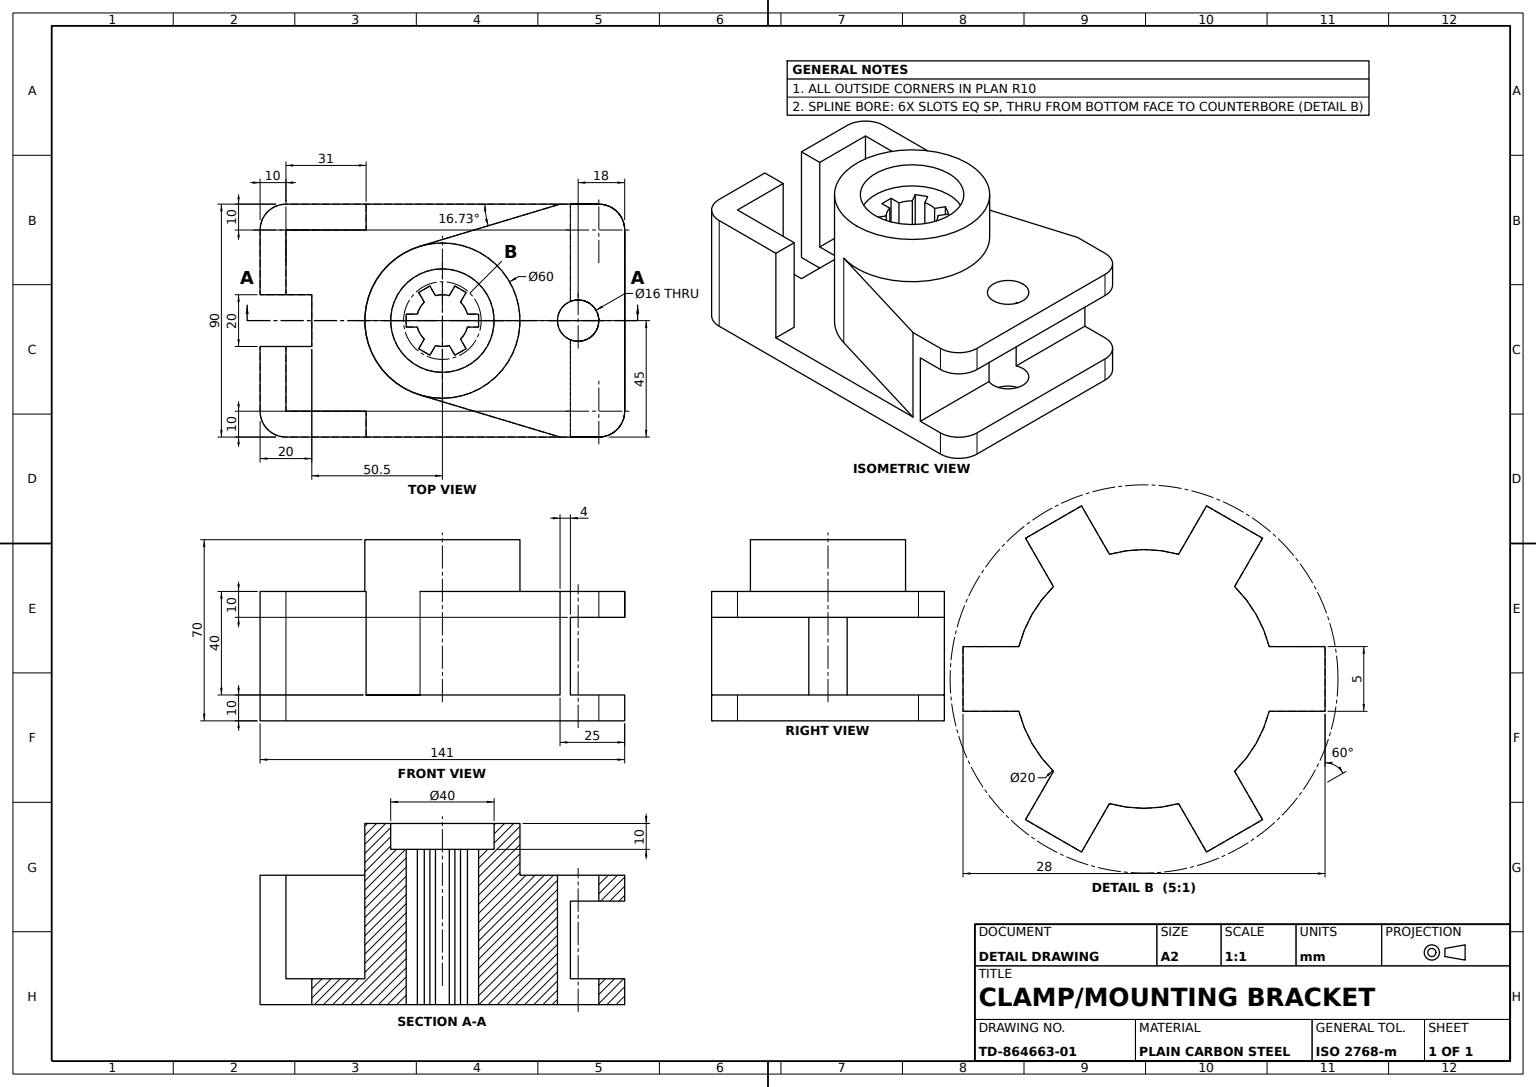
solid
v1 (0,70,20)
v2 (0,70,-20)
e1 v1 v2 CIRCLE(AX(P(0,70,0),D(0,1,0),D(0,0,1)),20)
e2 v2 v1 CIRCLE(AX(P(0,70,0),D(0,1,0),D(0,0,1)),20)
v3 (0,70,30)
v4 (0,70,-30)
e3 v3 v4 CIRCLE(AX(P(0,70,0),D(0,1,0),D(0,0,1)),30)
e4 v4 v3 CIRCLE(AX(P(0,70,0),D(0,1,0),D(0,0,1)),30)
face PLANE(AX(P(0,70,0),D(0,1,0),D(0,0,1))) [-e1 -e2] [e3 e4]
v5 (70.5,40,35)
v6 (70.5,40,-35)
e5 v5 v6 LINE
v7 (70.5,50,-35)
e6 v6 v7 LINE
v8 (70.5,50,35)
e7 v8 v7 LINE
e8 v5 v8 LINE
face PLANE(AX(P(70.5,40,-35),D(1,0,0),D(0,0,-1))) [e5 e6 -e7 -e8]
v9 (-7.006293,60,-7.135255)
v10 (-9.165064,60,-10.874356)
e9 v9 v10 LINE
v11 (-7.006293,0,-7.135255)
e10 v11 v9 LINE
v12 (-9.165064,0,-10.874356)
e11 v11 v12 LINE
e12 v12 v10 LINE
face PLANE(AX(P(-2.165064,-30,1.25),D(0.866025404,0,-0.5),D(-0.5,0,-0.866025404))) [-e9 -e10 e11 e12]
v13 (9.682458,60,2.5)
v14 (14,60,2.5)
e13 v13 v14 LINE
v15 (14,0,2.5)
e14 v15 v14 LINE
v16 (9.682458,0,2.5)
e15 v16 v15 LINE
e16 v16 v13 LINE
face PLANE(AX(P(0,-30,2.5),D(0,0,1),D(1,0,0))) rev [e13 -e14 -e15 e16]
v17 (70.5,10,35)
v18 (70.5,0,35)
e17 v17 v18 LINE
v19 (70.5,0,-35)
e18 v19 v18 LINE
v20 (70.5,10,-35)
e19 v20 v19 LINE
e20 v20 v17 LINE
face PLANE(AX(P(70.5,10,0),D(1,0,0),D(0,0,-1))) [e17 -e18 -e19 e20]
v21 (60.5,50,-45)
e21 v7 v21 CIRCLE(AX(P(60.5,50,-35),D(0,1,0),D(0,0,-1)),10)
v22 (60.5,40,-45)
e22 v6 v22 CIRCLE(AX(P(60.5,40,-35),D(0,1,0),D(0,0,-1)),10)
e23 v22 v21 LINE
face CYL(AX(P(60.5,40,-35),D(0,1,0),D(0,0,1)),10) [-e21 -e6 e22 e23]
v23 (49.5,10,-45)
v24 (49.5,10,-7.416198)
e24 v23 v24 LINE
v25 (52.5,10,-8)
e25 v25 v24 CIRCLE(AX(P(52.5,10,0),D(0,1,0),D(0,0,1)),8)
v26 (52.5,10,8)
e26 v26 v25 CIRCLE(AX(P(52.5,10,0),D(0,1,0),D(0,0,1)),8)
v27 (49.5,10,7.416198)
e27 v27 v26 CIRCLE(AX(P(52.5,10,0),D(0,1,0),D(0,0,1)),8)
v28 (49.5,10,45)
e28 v27 v28 LINE
v29 (60.5,10,45)
e29 v28 v29 LINE
e30 v29 v17 CIRCLE(AX(P(60.5,10,35),D(0,1,0),D(0,0,1)),10)
v30 (60.5,10,-45)
e31 v30 v20 CIRCLE(AX(P(60.5,10,-35),D(0,-1,0),D(0,0,1)),10)
e32 v23 v30 LINE
face PLANE(AX(P(0,10,0),D(0,1,0),D(0,0,1))) [e24 -e25 -e26 -e27 e28 e29 e30 -e20 -e31 -e32]
v31 (60.5,50,45)
e33 v31 v8 CIRCLE(AX(P(60.5,50,35),D(0,1,0),D(0,0,1)),10)
v32 (60.5,40,45)
e34 v32 v31 LINE
e35 v32 v5 CIRCLE(AX(P(60.5,40,35),D(0,1,0),D(0,0,1)),10)
face CYL(AX(P(60.5,40,35),D(0,1,0),D(0,0,1)),10) [e8 -e33 -e34 e35]
v33 (7.006293,60,7.135255)
v34 (9.165064,60,10.874356)
e36 v33 v34 LINE
v35 (7.006293,0,7.135255)
e37 v35 v33 LINE
v36 (9.165064,0,10.874356)
e38 v35 v36 LINE
e39 v36 v34 LINE
face PLANE(AX(P(2.165064,-30,-1.25),D(-0.866025404,0,0.5),D(0.5,0,0.866025404))) [-e36 -e37 e38 e39]
v37 (-60.5,10,-35)
v38 (-60.5,10,-10)
e40 v37 v38 LINE
v39 (-50.5,10,-10)
e41 v38 v39 LINE
v40 (-50.5,10,10)
e42 v40 v39 LINE
v41 (-60.5,10,10)
e43 v41 v40 LINE
v42 (-60.5,10,35)
e44 v42 v41 LINE
v43 (-29.5,10,35)
e45 v43 v42 LINE
v44 (-29.5,10,45)
e46 v44 v43 LINE
v45 (45.5,10,45)
e47 v44 v45 LINE
v46 (-8.634597,10,28.730537)
e48 v46 v45 LINE
v47 (-8.634597,10,-28.730537)
e49 v47 v46 CIRCLE(AX(P(0,10,0),D(0,1,0),D(0,0,1)),30)
v48 (45.5,10,-45)
e50 v48 v47 LINE
v49 (-29.5,10,-45)
e51 v49 v48 LINE
v50 (-29.5,10,-35)
e52 v49 v50 LINE
e53 v50 v37 LINE
face PLANE(AX(P(0,10,0),D(0,1,0),D(0,0,1))) [e40 e41 -e42 -e43 -e44 -e45 -e46 e47 -e48 -e49 -e50 -e51 e52 e53]
v51 (9.682458,0,-2.5)
v52 (9.682458,60,-2.5)
e54 v51 v52 LINE
v53 (7.006293,60,-7.135255)
e55 v52 v53 CIRCLE(AX(P(0,60,0),D(0,1,0),D(0,0,1)),10)
v54 (7.006293,0,-7.135255)
e56 v54 v53 LINE
e57 v51 v54 CIRCLE(AX(P(0,0,0),D(0,1,0),D(0,0,1)),10)
face CYL(AX(P(0,-30,0),D(0,1,0),D(0,0,1)),10) rev [e54 e55 -e56 -e57]
v55 (-29.5,50,35)
e58 v55 v43 LINE
v56 (-29.5,50,45)
e59 v56 v55 LINE
e60 v56 v44 LINE
face PLANE(AX(P(-29.5,50,0),D(-1,0,0),D(0,0,1))) rev [e46 -e58 -e59 e60]
v57 (-2.676166,0,-9.635255)
v58 (-4.834936,0,-13.374356)
e61 v57 v58 LINE
v59 (-2.676166,60,-9.635255)
e62 v57 v59 LINE
v60 (-4.834936,60,-13.374356)
e63 v59 v60 LINE
e64 v58 v60 LINE
face PLANE(AX(P(2.165064,-30,-1.25),D(0.866025404,0,-0.5),D(-0.5,0,-0.866025404))) rev [-e61 e62 e63 -e64]
v61 (0,50,30)
e65 v3 v61 LINE
v62 (0,50,-30)
e66 v62 v61 CIRCLE(AX(P(0,50,0),D(0,-1,0),D(0,0,1)),30)
e67 v4 v62 LINE
face CYL(AX(P(0,50,0),D(0,-1,0),D(0,0,-1)),30) [e65 -e66 -e67 -e3]
v63 (-14,0,-2.5)
v64 (-14,60,-2.5)
e68 v63 v64 LINE
v65 (-14,60,2.5)
e69 v65 v64 LINE
v66 (-14,0,2.5)
e70 v66 v65 LINE
e71 v66 v63 LINE
face PLANE(AX(P(-14,-30,0),D(1,0,0),D(0,0,-1))) [e68 -e69 -e70 e71]
v67 (60.5,0,-45)
e72 v67 v19 CIRCLE(AX(P(60.5,0,-35),D(0,-1,0),D(0,0,1)),10)
e73 v30 v67 LINE
face CYL(AX(P(60.5,10,-35),D(0,-1,0),D(0,0,-1)),10) [e19 -e72 -e73 e31]
v68 (-60.5,50,-35)
v69 (-60.5,50,-10)
e74 v68 v69 LINE
e75 v69 v38 LINE
e76 v68 v37 LINE
face PLANE(AX(P(-60.5,50,0),D(1,0,0),D(0,0,-1))) [e74 e75 -e40 -e76]
v70 (52.5,40,-8)
v71 (52.5,50,-8)
e77 v70 v71 LINE
v72 (52.5,40,8)
e78 v70 v72 CIRCLE(AX(P(52.5,40,0),D(0,-1,0),D(0,0,-1)),8)
v73 (52.5,50,8)
e79 v72 v73 LINE
e80 v73 v71 CIRCLE(AX(P(52.5,50,0),D(0,1,0),D(0,0,1)),8)
face CYL(AX(P(52.5,-40,0),D(0,1,0),D(0,0,1)),8) rev [-e77 e78 e79 e80]
v74 (-70.5,50,-10)
e81 v74 v69 LINE
v75 (-70.5,0,-10)
e82 v74 v75 LINE
v76 (-50.5,0,-10)
e83 v75 v76 LINE
e84 v39 v76 LINE
face PLANE(AX(P(0,10,-10),D(0,0,-1),D(-1,0,0))) rev [-e81 e82 e83 -e84 -e41 -e75]
v77 (-4.834936,0,13.374356)
v78 (-4.834936,60,13.374356)
e85 v77 v78 LINE
v79 (-2.676166,60,9.635255)
e86 v78 v79 LINE
v80 (-2.676166,0,9.635255)
e87 v80 v79 LINE
e88 v77 v80 LINE
face PLANE(AX(P(2.165064,-30,1.25),D(0.866025404,0,0.5),D(0.5,0,-0.866025404))) rev [e85 e86 -e87 -e88]
v81 (2.676166,0,9.635255)
v82 (2.676166,60,9.635255)
e89 v81 v82 LINE
v83 (4.834936,60,13.374356)
e90 v82 v83 LINE
v84 (4.834936,0,13.374356)
e91 v84 v83 LINE
e92 v81 v84 LINE
face PLANE(AX(P(-2.165064,-30,1.25),D(-0.866025404,0,0.5),D(0.5,0,0.866025404))) rev [e89 e90 -e91 -e92]
v85 (-60.5,50,35)
e93 v55 v85 LINE
v86 (-60.5,50,10)
e94 v85 v86 LINE
v87 (-70.5,50,10)
e95 v86 v87 LINE
v88 (-70.5,50,35)
e96 v87 v88 LINE
v89 (-60.5,50,45)
e97 v88 v89 CIRCLE(AX(P(-60.5,50,35),D(0,1,0),D(0,0,1)),10)
e98 v89 v56 LINE
face PLANE(AX(P(0,50,0),D(0,1,0),D(0,0,1))) [e59 e93 e94 e95 e96 e97 e98]
v90 (52.5,0,-8)
e99 v90 v25 LINE
v91 (52.5,0,8)
e100 v91 v90 CIRCLE(AX(P(52.5,0,0),D(0,1,0),D(0,0,1)),8)
e101 v91 v26 LINE
face CYL(AX(P(52.5,-40,0),D(0,1,0),D(0,0,1)),8) rev [-e99 -e100 e101 e26]
e102 v35 v16 CIRCLE(AX(P(0,0,0),D(0,1,0),D(0,0,1)),10)
e103 v33 v13 CIRCLE(AX(P(0,60,0),D(0,1,0),D(0,0,1)),10)
face CYL(AX(P(0,-30,0),D(0,1,0),D(0,0,1)),10) rev [-e102 e37 e103 -e16]
v92 (49.5,40,45)
e104 v28 v92 LINE
v93 (49.5,40,7.416198)
e105 v93 v27 LINE
e106 v93 v92 LINE
face PLANE(AX(P(49.5,50,-45),D(1,0,0),D(0,0,-1))) [-e104 -e28 -e105 e106]
v94 (0,60,20)
e107 v94 v1 LINE
v95 (0,60,-20)
e108 v95 v94 CIRCLE(AX(P(0,60,0),D(0,1,0),D(0,0,1)),20)
e109 v95 v2 LINE
face CYL(AX(P(0,60,0),D(0,1,0),D(0,0,1)),20) rev [e2 -e107 -e108 e109]
e110 v36 v84 LINE
e111 v34 v83 LINE
face PLANE(AX(P(7,-30,12.124356),D(-0.5,0,-0.866025404),D(-0.866025404,0,0.5))) [e110 e91 -e111 -e39]
v96 (2.676166,0,-9.635255)
v97 (2.676166,60,-9.635255)
e112 v96 v97 LINE
v98 (4.834936,0,-13.374356)
e113 v96 v98 LINE
v99 (4.834936,60,-13.374356)
e114 v98 v99 LINE
e115 v97 v99 LINE
face PLANE(AX(P(-2.165064,-30,-1.25),D(0.866025404,0,0.5),D(0.5,0,-0.866025404))) [-e112 e113 e114 -e115]
v100 (45.5,50,45)
e116 v100 v45 LINE
v101 (-8.634597,50,28.730537)
e117 v101 v100 LINE
e118 v101 v46 LINE
face PLANE(AX(P(-8.634597,50,28.730537),D(0.287819891,0,-0.957684557),D(-0.957684557,0,-0.287819891))) rev [-e116 -e117 e118 e48]
v102 (45.5,50,-45)
e119 v102 v48 LINE
e120 v21 v102 LINE
v103 (49.5,40,-45)
e121 v22 v103 LINE
e122 v23 v103 LINE
v104 (-60.5,0,-45)
e123 v104 v67 LINE
v105 (-60.5,50,-45)
e124 v105 v104 LINE
v106 (-29.5,50,-45)
e125 v106 v105 LINE
e126 v106 v49 LINE
face PLANE(AX(P(0,10,-45),D(0,0,-1),D(-1,0,0))) [e51 -e119 -e120 -e23 e121 -e122 e32 e73 -e123 -e124 -e125 e126]
v107 (-70.5,0,10)
e127 v87 v107 LINE
v108 (-70.5,0,35)
e128 v107 v108 LINE
e129 v88 v108 LINE
face PLANE(AX(P(-70.5,10,0),D(1,0,0),D(0,0,-1))) rev [e127 e128 -e129 -e96]
e130 v94 v95 CIRCLE(AX(P(0,60,0),D(0,1,0),D(0,0,1)),20)
face CYL(AX(P(0,60,0),D(0,1,0),D(0,0,1)),20) rev [e107 e1 -e109 -e130]
v109 (-8.634597,50,-28.730537)
e131 v109 v62 CIRCLE(AX(P(0,50,0),D(0,-1,0),D(0,0,1)),30)
e132 v61 v101 CIRCLE(AX(P(0,50,0),D(0,-1,0),D(0,0,1)),30)
e133 v100 v31 LINE
e134 v102 v109 LINE
e135 v71 v73 CIRCLE(AX(P(52.5,50,0),D(0,1,0),D(0,0,1)),8)
face PLANE(AX(P(0,50,0),D(0,1,0),D(0,0,1))) [e131 e66 e132 e117 e133 e33 e7 e21 e120 e134] [-e135 -e80]
v110 (49.5,40,-7.416198)
e136 v24 v110 LINE
e137 v103 v110 LINE
face PLANE(AX(P(49.5,50,-45),D(1,0,0),D(0,0,-1))) [-e136 -e24 e122 e137]
v111 (60.5,0,45)
e138 v111 v18 CIRCLE(AX(P(60.5,0,35),D(0,1,0),D(0,0,1)),10)
e139 v29 v111 LINE
face CYL(AX(P(60.5,10,35),D(0,-1,0),D(0,0,-1)),10) [e138 -e17 -e30 e139]
v112 (9.165064,60,-10.874356)
e140 v53 v112 LINE
v113 (9.165064,0,-10.874356)
e141 v113 v112 LINE
e142 v54 v113 LINE
face PLANE(AX(P(2.165064,-30,1.25),D(0.866025404,0,0.5),D(0.5,0,-0.866025404))) rev [e140 -e141 -e142 e56]
v114 (-50.5,0,10)
e143 v114 v76 LINE
e144 v40 v114 LINE
face PLANE(AX(P(-50.5,10,0),D(-1,0,0),D(0,0,1))) [e84 -e143 -e144 e42]
v115 (-29.5,50,-35)
e145 v115 v68 LINE
e146 v115 v50 LINE
face PLANE(AX(P(0,50,-35),D(0,0,1),D(1,0,0))) [e145 e76 -e53 -e146]
v116 (-9.682458,0,2.5)
v117 (-9.682458,60,2.5)
e147 v116 v117 LINE
v118 (-7.006293,60,7.135255)
e148 v117 v118 CIRCLE(AX(P(0,60,0),D(0,1,0),D(0,0,1)),10)
v119 (-7.006293,0,7.135255)
e149 v119 v118 LINE
e150 v116 v119 CIRCLE(AX(P(0,0,0),D(0,1,0),D(0,0,1)),10)
face CYL(AX(P(0,-30,0),D(0,1,0),D(0,0,1)),10) rev [e147 e148 -e149 -e150]
e151 v109 v47 LINE
face PLANE(AX(P(-8.634597,50,-28.730537),D(0.287819891,0,0.957684557),D(0.957684557,0,-0.287819891))) rev [-e134 e119 e50 -e151]
e152 v90 v91 CIRCLE(AX(P(52.5,0,0),D(0,1,0),D(0,0,1)),8)
v120 (-60.5,0,45)
e153 v120 v111 LINE
e154 v108 v120 CIRCLE(AX(P(-60.5,0,35),D(0,1,0),D(0,0,1)),10)
e155 v107 v114 LINE
v121 (-70.5,0,-35)
e156 v121 v75 LINE
e157 v104 v121 CIRCLE(AX(P(-60.5,0,-35),D(0,1,0),D(0,0,1)),10)
v122 (-9.165064,0,10.874356)
e158 v77 v122 LINE
v123 (0,0,10)
e159 v80 v123 CIRCLE(AX(P(0,0,0),D(0,1,0),D(0,0,1)),10)
e160 v123 v81 CIRCLE(AX(P(0,0,0),D(0,1,0),D(0,0,1)),10)
v124 (14,0,-2.5)
e161 v124 v15 LINE
e162 v51 v124 LINE
e163 v98 v113 LINE
e164 v96 v57 CIRCLE(AX(P(0,0,0),D(0,1,0),D(0,0,1)),10)
e165 v12 v58 LINE
v125 (-9.682458,0,-2.5)
e166 v11 v125 CIRCLE(AX(P(0,0,0),D(0,1,0),D(0,0,1)),10)
e167 v125 v63 LINE
e168 v116 v66 LINE
e169 v119 v122 LINE
face PLANE(AX(P(0,0,0),D(0,1,0),D(0,0,1))) rev [e152 e100] [e72 e18 -e138 -e153 -e154 -e128 e155 e143 -e83 -e156 -e157 e123] [-e158 e88 e159 e160 e92 -e110 -e38 e102 e15 -e161 -e162 e57 e142 -e163 -e113 e164 e61 -e165 -e11 e166 e167 -e71 -e168 e150 e169]
e170 v117 v65 LINE
face PLANE(AX(P(0,-30,2.5),D(0,0,-1),D(-1,0,0))) [e70 -e170 -e147 e168]
v126 (0,60,10)
e171 v123 v126 LINE
e172 v126 v82 CIRCLE(AX(P(0,60,0),D(0,1,0),D(0,0,1)),10)
face CYL(AX(P(0,-30,0),D(0,1,0),D(0,0,1)),10) rev [-e89 -e160 e171 e172]
v127 (-9.165064,60,10.874356)
e173 v122 v127 LINE
e174 v78 v127 LINE
face PLANE(AX(P(-7,-30,12.124356),D(0.5,0,-0.866025404),D(-0.866025404,0,-0.5))) [-e85 e158 e173 -e174]
e175 v89 v120 LINE
face CYL(AX(P(-60.5,10,35),D(0,-1,0),D(0,0,-1)),10) [-e97 e129 e154 -e175]
v128 (-70.5,50,-35)
e176 v128 v121 LINE
e177 v105 v128 CIRCLE(AX(P(-60.5,50,-35),D(0,1,0),D(0,0,1)),10)
face CYL(AX(P(-60.5,10,-35),D(0,-1,0),D(0,0,-1)),10) [-e176 -e177 e124 e157]
e178 v86 v41 LINE
face PLANE(AX(P(0,10,10),D(0,0,-1),D(-1,0,0))) [-e155 -e127 -e95 e178 e43 e144]
e179 v85 v42 LINE
face PLANE(AX(P(-60.5,50,0),D(-1,0,0),D(0,0,1))) rev [-e178 -e94 e179 e44]
e180 v97 v59 CIRCLE(AX(P(0,60,0),D(0,1,0),D(0,0,1)),10)
face CYL(AX(P(0,-30,0),D(0,1,0),D(0,0,1)),10) rev [-e164 e112 e180 -e62]
e181 v92 v32 LINE
face PLANE(AX(P(0,10,45),D(0,0,-1),D(-1,0,0))) rev [e104 e181 e34 -e133 e116 -e47 -e60 -e98 e175 e153 -e139 -e29]
e182 v79 v126 CIRCLE(AX(P(0,60,0),D(0,1,0),D(0,0,1)),10)
face CYL(AX(P(0,-30,0),D(0,1,0),D(0,0,1)),10) rev [-e159 e87 e182 -e171]
e183 v99 v112 LINE
face PLANE(AX(P(7,-30,-12.124356),D(-0.5,0,0.866025404),D(0.866025404,0,0.5))) [e163 e141 -e183 -e114]
e184 v106 v115 LINE
face PLANE(AX(P(-29.5,50,0),D(1,0,0),D(0,0,-1))) [-e126 e184 e146 -e52]
e185 v72 v93 CIRCLE(AX(P(52.5,40,0),D(0,-1,0),D(0,0,-1)),8)
e186 v110 v70 CIRCLE(AX(P(52.5,40,0),D(0,-1,0),D(0,0,-1)),8)
face PLANE(AX(P(60.5,40,-35),D(0,-1,0),D(0,0,-1))) [-e22 -e5 -e35 -e181 -e106 -e185 -e78 -e186 -e137 -e121]
e187 v128 v74 LINE
face PLANE(AX(P(0,50,0),D(0,1,0),D(0,0,1))) [e187 e81 -e74 -e145 -e184 e125 e177]
face CYL(AX(P(0,50,0),D(0,-1,0),D(0,0,-1)),30) [e151 e49 -e118 -e132 -e65 -e4 e67 -e131]
v129 (-9.682458,60,-2.5)
e188 v125 v129 LINE
e189 v129 v64 LINE
face PLANE(AX(P(0,-30,-2.5),D(0,0,-1),D(-1,0,0))) rev [e188 e189 -e68 -e167]
e190 v118 v127 LINE
face PLANE(AX(P(-2.165064,-30,-1.25),D(-0.866025404,0,-0.5),D(-0.5,0,0.866025404))) rev [-e169 e149 e190 -e173]
v130 (14,60,-2.5)
e191 v130 v14 LINE
e192 v124 v130 LINE
face PLANE(AX(P(14,-30,0),D(-1,0,0),D(0,0,1))) [e161 e14 -e191 -e192]
face PLANE(AX(P(0,50,35),D(0,0,1),D(1,0,0))) rev [e45 -e179 -e93 e58]
e193 v10 v60 LINE
face PLANE(AX(P(-7,-30,-12.124356),D(0.5,0,0.866025404),D(0.866025404,0,-0.5))) [-e193 -e12 e165 e64]
face PLANE(AX(P(-70.5,10,0),D(1,0,0),D(0,0,-1))) rev [-e82 -e187 e176 e156]
face CYL(AX(P(52.5,-40,0),D(0,1,0),D(0,0,1)),8) rev [e25 e136 e186 e77 e135 -e79 e185 e105 e27 -e101 -e152 e99]
e194 v9 v129 CIRCLE(AX(P(0,60,0),D(0,1,0),D(0,0,1)),10)
e195 v52 v130 LINE
face PLANE(AX(P(0,60,0),D(0,1,0),D(0,0,1))) [e130 e108] [e36 e111 -e90 -e172 -e182 -e86 e174 -e190 -e148 e170 e69 -e189 -e194 e9 e193 -e63 -e180 e115 e183 -e140 -e55 e195 e191 -e13 -e103]
face CYL(AX(P(0,-30,0),D(0,1,0),D(0,0,1)),10) rev [e194 -e188 -e166 e10]
face PLANE(AX(P(0,-30,-2.5),D(0,0,1),D(1,0,0))) [e162 e192 -e195 -e54]
